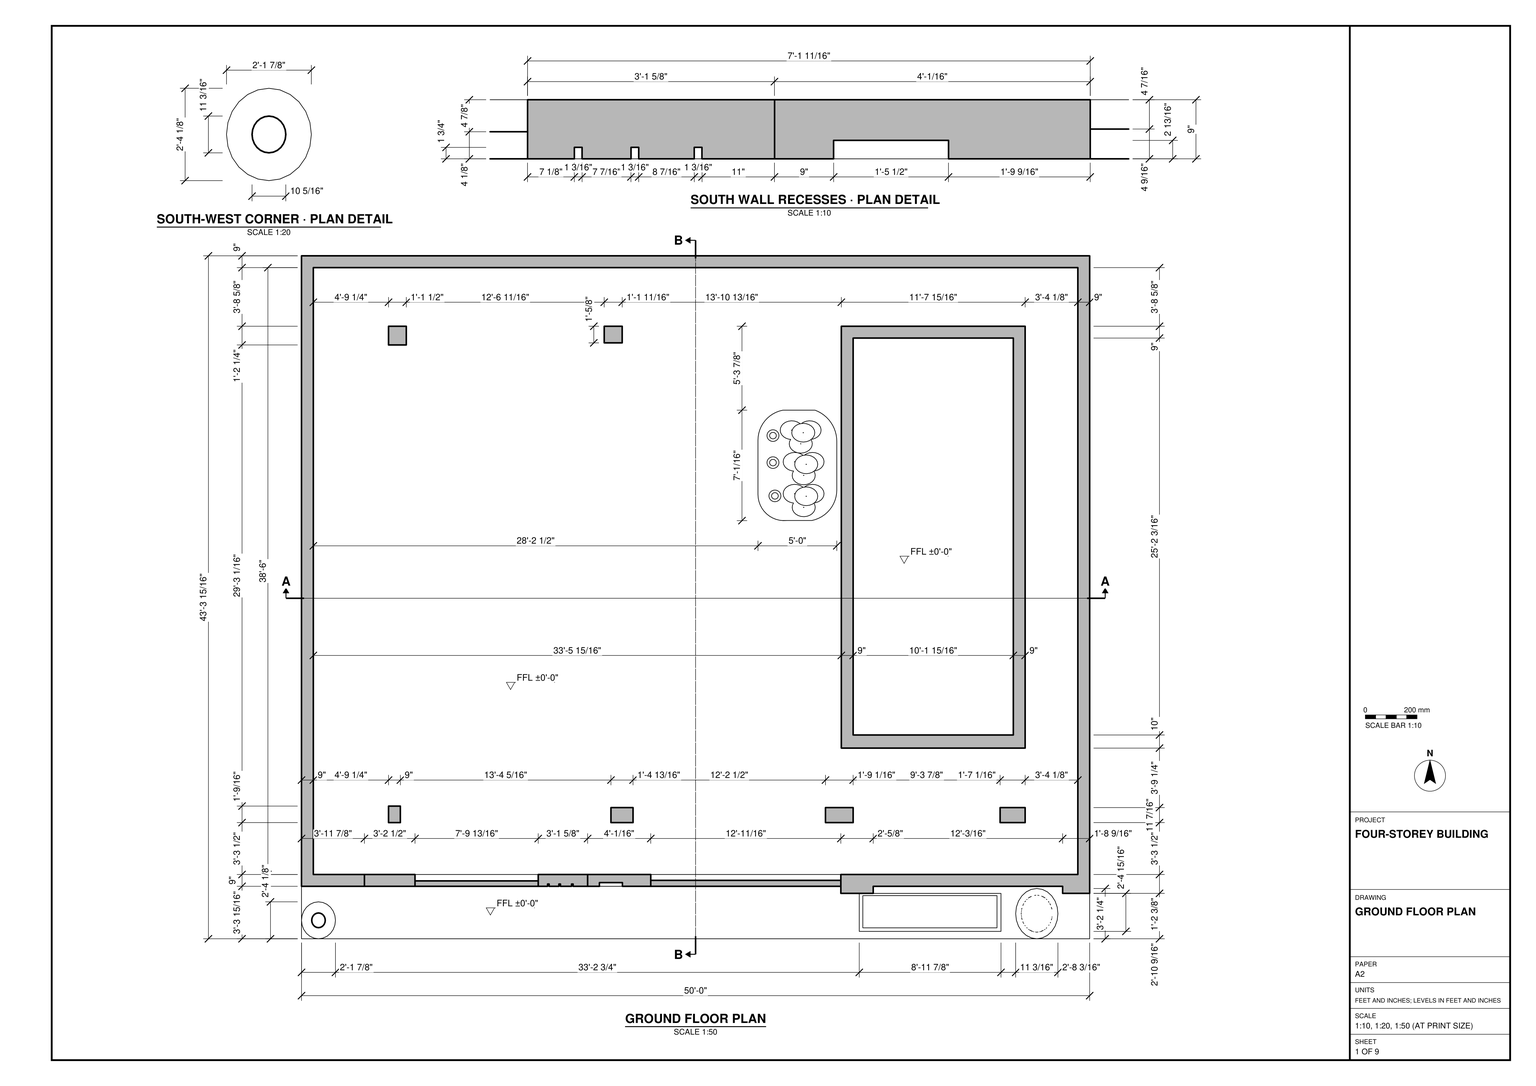
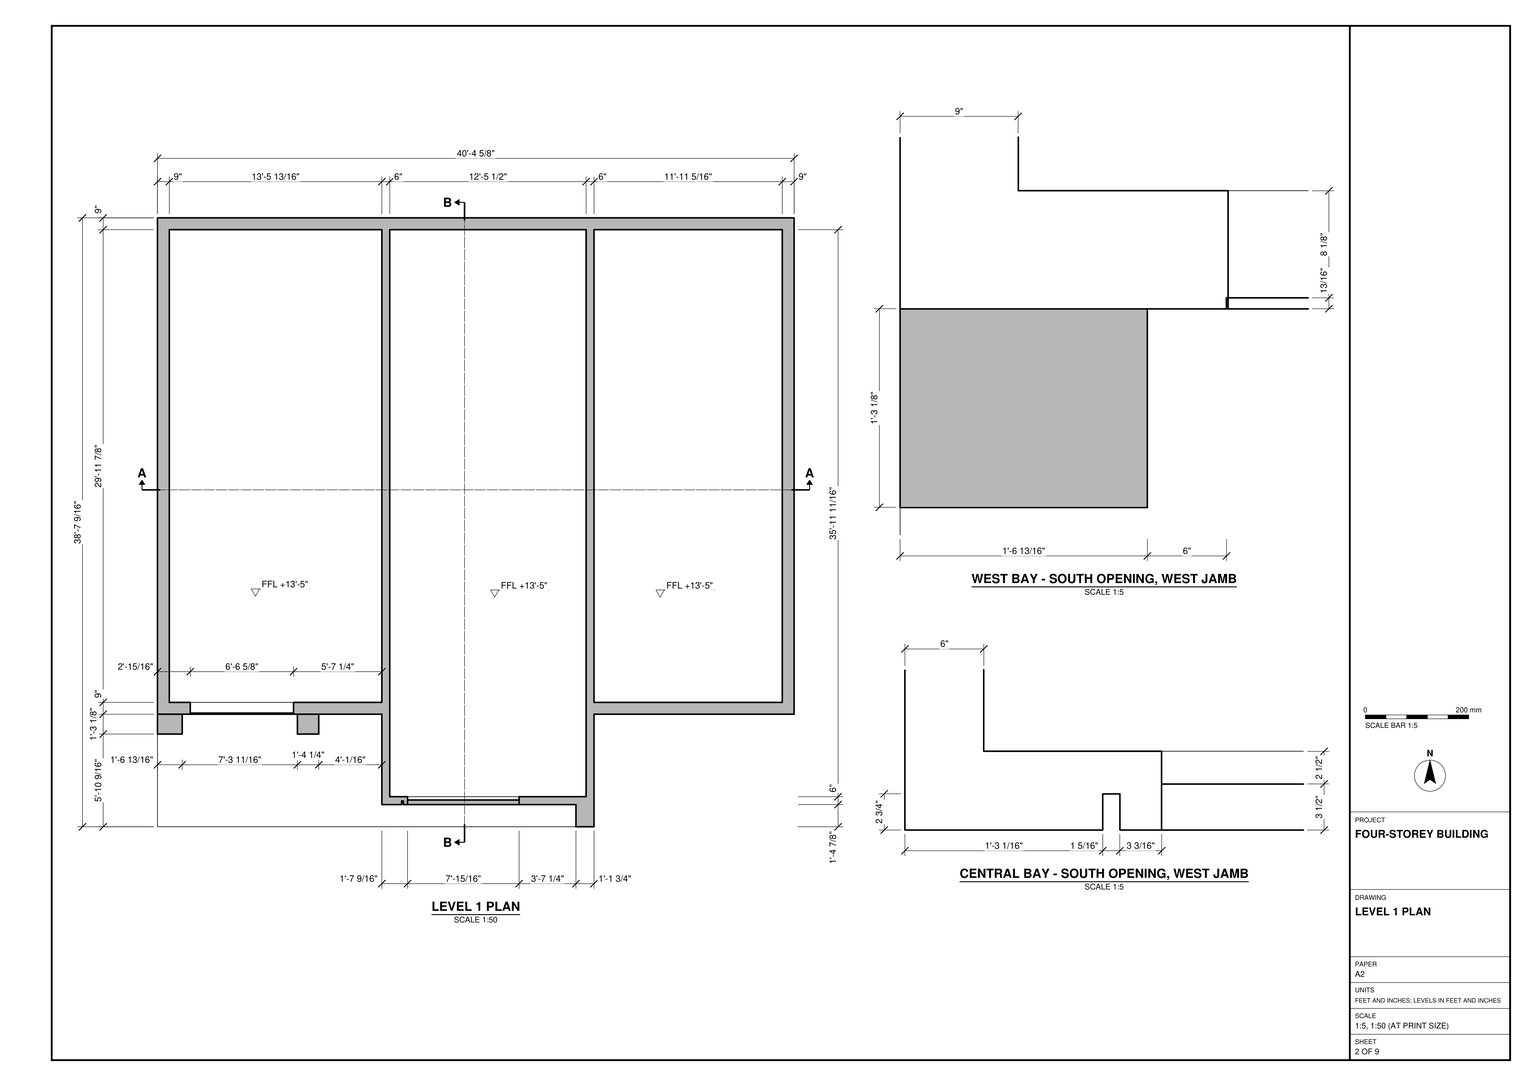
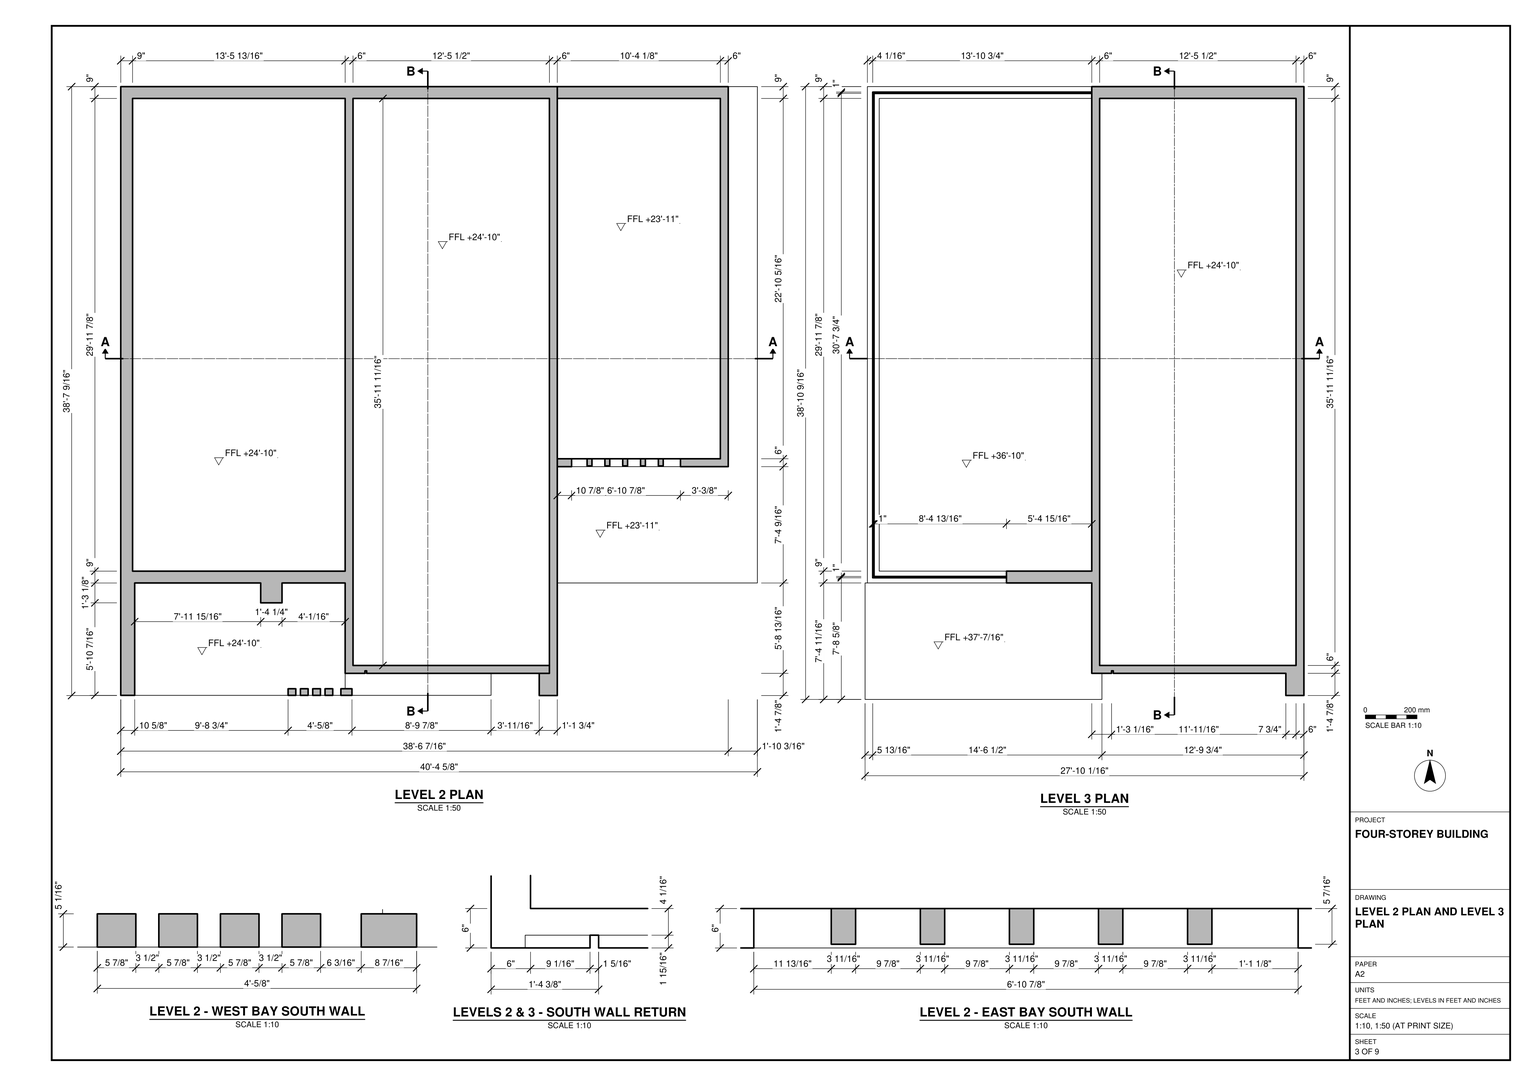
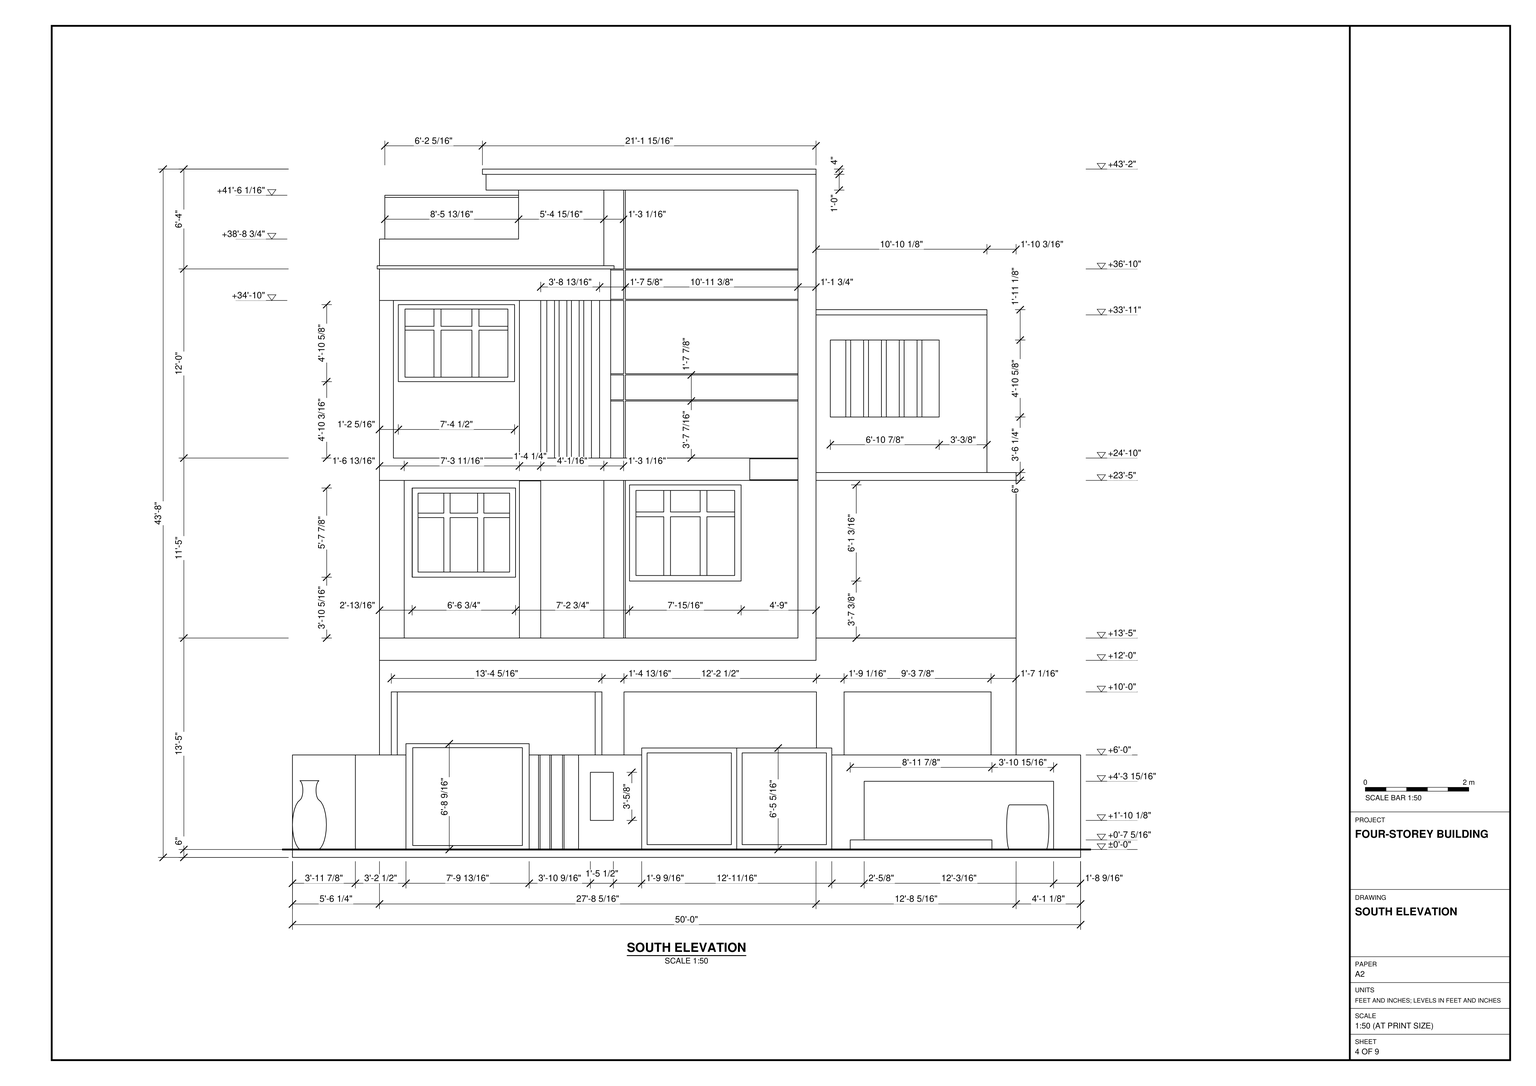
Build the four-storey building in SketchUp from task_files/diagram_01.pdf. Work in feet and inches. The overall size is 50'-0" east to west, 43'-5 7/16" north to south and 43'-8" high. Set the main floor levels at ±0'-0", +13'-5", +24'-10" and +36'-10". Follow the local changes in floor and roof height shown on the sheets rather than levelling each slab across all bays.

Lay out the largely open ground floor with its freestanding columns, long rectangular enclosure near the east side and narrow strip beyond the south wall. Use the plan details for the recesses in that wall. Above it, form the three north–south bays, with the central bay projecting farther south than the side bays. Follow the changes in footprint on the upper floors, including the setback of the east bay. Use the wall thicknesses shown, including the 9" perimeter walls and 6" dividing walls where dimensioned. Model the openings and jambs, floor slabs, exposed roof areas and roof edges from the plans and sections. Include stairs, built-in joinery and main furniture where shown.

Keep walls, slabs, roof elements and each furniture or joinery piece in separate groups or components. Use components for repeated parts. Decor and loose items may be any suitable library components. Save one SketchUp model as output_files/four_storey_building_with_stepped_upper_bays.skp.

# SketchUp Ruby script. Lengths in inches.
U = 1.inch
M = Sketchup.active_model
def pt(a) = Geom::Point3d.new(a.map { |v| v * U })
def face(e, loops, mat)
  f = e.add_face(loops[0].map { |a| pt(a) })
  loops[1..].each { |l| e.add_face(l.map { |a| pt(a) }).erase! }
  f.material = f.back_material = mat if mat
  f
end
# faces: each face lists its corners as indices into pts; further lists are holes
def faces(e, pts, list, mat = nil) = list.each { |f| face(e, (f[0].is_a?(Array) ? f : [f]).map { |l| l.map { |i| pts[i] } }, mat) }
# xy, xz, yz: faces in a plane at the given z, y or x. An outline is a flat list of corners, or four numbers for a rectangle; further outlines are holes
def ring(l) = l.size == 4 ? [[l[0], l[1]], [l[2], l[1]], [l[2], l[3]], [l[0], l[3]]] : l.each_slice(2).to_a
def flat(e, list, mat, &to3) = list.each { |f| face(e, (f[0].is_a?(Array) ? f : [f]).map { |l| ring(l).map { |u, v| to3.(u, v) } }, mat) }
def xy(e, z, list, mat = nil) = flat(e, list, mat) { |x, y| [x, y, z] }
def xz(e, y, list, mat = nil) = flat(e, list, mat) { |x, z| [x, y, z] }
def yz(e, x, list, mat = nil) = flat(e, list, mat) { |y, z| [x, y, z] }
def lines(e, pts, list) = list.each { |a, b| e.add_line(pt(pts[a]), pt(pts[b])) }
# prism: a flat outline (further loops are holes) pulled along v
def prism(e, loops, v, mat = nil)
  f = face(e, loops, mat); d = Geom::Vector3d.new(v.map { |x| x * U })
  f.pushpull(f.normal.samedirection?(d) ? d.length : -d.length)
end
def box(e, o, s, mat = nil) = prism(e, [[o, [o[0] + s[0], o[1], o[2]], [o[0] + s[0], o[1] + s[1], o[2]], [o[0], o[1] + s[1], o[2]]]], [0, 0, s[2]], mat)
def at(x, y, z, deg = 0) = Geom::Transformation.translation(pt([x, y, z])) * Geom::Transformation.rotation(ORIGIN, Z_AXIS, deg.degrees)
def axes(o, x, y, z) = Geom::Transformation.new([*x, 0, *y, 0, *z, 0, *pt(o).to_a, 1])
def part(name) = M.definitions.add(name)
# library, detail: a bought-in or finely detailed component or shape, given as its bounding box
def library(name, o, s) = part(name).tap { |d| box(d.entities, o, s) }
def detail(e, o, s) = box(e.add_group.entities, o, s)
def put(e, d, t, mat = nil) = e.add_instance(d, t).tap { |i| i.material = mat if mat }
def group(e, t, mat = nil) = e.add_group.tap { |g| g.transformation = t; g.material = mat if mat }.entities
root = M.entities
M.materials.add("[0056_Yellow]").color = [249, 242, 89]
M.materials.add("[0056_Yellow]1").color = [255, 255, 0]
M.materials.add("[0060_GrassGreen]").color = [62, 91, 76]
M.materials.add("[0073_MediumSeaGreen]").color = [60, 179, 113]
M.materials.add("[0111_SlateGray]").color = [120, 130, 144]
M.materials.add("[0123_DarkMagenta]").color = [145, 113, 139]
M.materials.add("[0124_Purple]").color = [128, 93, 128]
M.materials.add("[0131_Silver]").color = [192, 192, 192]
M.materials.add("[0136_Charcoal]").color = [35, 35, 35]
M.materials.add("[Brick Rough Tan]").color = [199, 186, 164]
M.materials.add("[Brick Rough Tan]1").color = [167, 141, 82]
M.materials.add("[Carrera Marble]").color = [207, 207, 207]
M.materials.add("[Color C08]").color = [102, 51, 0]
M.materials.add("[Color I01]").color = [204, 204, 255]
M.materials.add("[Color I06]").color = [0, 130, 204]
M.materials.add("[Color M00]").color = [255, 255, 255]
M.materials.add("[Color M01]").color = [226, 226, 226]
M.materials.add("[Color M02]").color = [198, 198, 198]
M.materials.add("[Color M03]").color = [170, 170, 170]
M.materials.add("[Color M04]").color = [142, 142, 142]
M.materials.add("[Color M06]").color = [86, 86, 86]
M.materials.add("[Color M07]").color = [58, 58, 58]
M.materials.add("[Concrete Block 8x8 Gray]").color = [157, 158, 154]
M.materials.add("[Concrete Block Retaining Gray]").color = [121, 121, 121]
M.materials.add("[Grass Dark Green]").color = [106, 157, 55]
M.materials.add("[Polished Concrete New]").color = [200, 200, 203]
M.materials.add("[Stone Flagstone Ashlar]").color = [106, 69, 26]
M.materials.add("[Translucent Glass Gray]").color = [128, 128, 128]
M.materials["[Translucent Glass Gray]"].alpha = 0.5
M.materials.add("[Wood Cherry Original]").color = [152, 86, 42]
M.materials.add("[Wood Floor Parquet]").color = [145, 89, 39]
c1 = part("Group\#1")
xy(c1.entities,0,[[0,0,56.875,3.5]],"[Wood Cherry Original]")
xy(c1.entities,3.27,[[3.27,0,17.44,3.5],[17.44,0,20.89,1.125],[20.89,0,36,3.5],[36,0,39.45,1.125],[39.45,0,53.6,3.5],
  [17.44,1.125,20.89,3.5],[36,1.125,39.45,3.5]],"[Wood Cherry Original]")
xy(c1.entities,38.03,[[3.27,1.125,17.44,3.5],[20.89,1.125,36,3.5],[39.45,1.125,53.6,3.5]],"[Wood Cherry Original]")
xy(c1.entities,40.86,[[3.27,1.125,17.44,3.5],[20.89,1.125,36,3.5],[39.45,1.125,53.6,3.5]],"[Wood Cherry Original]")
xy(c1.entities,53.6,[[3.27,0,17.44,3.5],[17.44,0,20.89,1.125],[20.89,0,36,3.5],[36,0,39.45,1.125],[39.45,0,53.6,3.5],
  [17.44,1.125,20.89,3.5],[36,1.125,39.45,3.5]],"[Wood Cherry Original]")
xy(c1.entities,56.875,[[0,0,56.875,3.5]],"[Wood Cherry Original]")
xz(c1.entities,0,[[[0,0,56.875,56.875],[3.27,3.27,53.6,53.6]]],"[Wood Cherry Original]")
xz(c1.entities,1.125,[[17.44,3.27,20.89,3.27,20.89,38.03,36,38.03,36,3.27,39.45,3.27,39.45,38.03,53.6,38.03,53.6,40.86,39.45,40.86,39.45,53.6,36,53.6,36,40.86,20.89,40.86,20.89,53.6,17.44,53.6,17.44,40.86,3.27,40.86,3.27,38.03,17.44,38.03]],"[Wood Cherry Original]")
xz(c1.entities,3.5,[[3.27,3.27,17.44,38.03],[20.89,3.27,36,38.03],[39.45,3.27,53.6,38.03],[3.27,40.86,17.44,53.6],[20.89,40.86,36,53.6],
  [39.45,40.86,53.6,53.6]],"[Translucent Glass Gray]")
xz(c1.entities,3.5,[[[0,0,56.875,56.875],[3.27,3.27,53.6,53.6]],[17.44,3.27,17.44,38.03,3.27,38.03,3.27,40.86,17.44,40.86,17.44,53.6,20.89,53.6,20.89,40.86,36,40.86,36,53.6,39.45,53.6,39.45,40.86,53.6,40.86,53.6,38.03,39.45,38.03,39.45,3.27,36,3.27,36,38.03,20.89,38.03,20.89,3.27]],"[Wood Cherry Original]")
yz(c1.entities,0,[[0,0,3.5,56.875]],"[Wood Cherry Original]")
yz(c1.entities,3.27,[[0,3.27,3.5,38.03],[0,38.03,1.125,40.86],[1.125,38.03,3.5,40.86],[0,40.86,3.5,53.6]],"[Wood Cherry Original]")
yz(c1.entities,17.44,[[1.125,3.27,3.5,38.03],[1.125,40.86,3.5,53.6]],"[Wood Cherry Original]")
yz(c1.entities,20.89,[[1.125,3.27,3.5,38.03],[1.125,40.86,3.5,53.6]],"[Wood Cherry Original]")
yz(c1.entities,36,[[1.125,3.27,3.5,38.03],[1.125,40.86,3.5,53.6]],"[Wood Cherry Original]")
yz(c1.entities,39.45,[[1.125,3.27,3.5,38.03],[1.125,40.86,3.5,53.6]],"[Wood Cherry Original]")
yz(c1.entities,53.6,[[0,3.27,3.5,38.03],[0,38.03,1.125,40.86],[1.125,38.03,3.5,40.86],[0,40.86,3.5,53.6]],"[Wood Cherry Original]")
yz(c1.entities,56.875,[[0,0,3.5,56.875]],"[Wood Cherry Original]")
c2 = library("Group\#4",[0,0,0],[25.84,28.11,66.36])
c3 = library("Group\#6",[0,0,0],[80.96,80.52,80.96])
c4 = library("Group\#7",[0,0,0],[79.77,94.6,79.77])
c5 = part("Group\#8")
xy(c5.entities,0,[[0.19,0.27,3.22,4.42]])
xy(c5.entities,14.6875,[[0,0,2.48,3.02]])
p = [[3.22,0.27,0],[2.48,0,14.6875],[0,0,14.6875],[0.19,0.27,0],[0,3.02,14.6875],[0.19,4.42,0],
  [3.22,4.42,0],[2.48,3.02,14.6875]]
faces(c5.entities,p,[[0,1,2,3],[2,4,5,3],[1,0,6,7],[5,4,7,6]])
c6 = library("Group\#10",[0,0,0],[17.53,14.22,10.22])
c7 = library("Group\#11",[0,0,0],[7.07,6.58,13.6])
xy(root,0,[[0,1.5,600,41.4375],[0,41.4375,600,521.4375]])
xy(root,6,[[410.58,36.0625,435.23,41.4375],[0,41.4375,0,521.4375,600,521.4375,600,41.4375,410.58,41.4375,410.58,50.4375,591,50.4375,591,512.4375,9,512.4375,9,50.4375,47.9,50.4375,47.9,41.4375],[47.9,41.4375,86.4,50.4375],[86.4,41.4375,180.2,50.4375],[180.2,41.4375,180.2,50.4375,217.8125,50.4375,217.8125,41.4375,206.75,41.4375,206.75,43.1875,205.58,43.1875,205.58,41.4375,197.125,41.4375,197.125,43.1875,195.95,43.1875,195.95,41.4375,188.5,41.4375,188.5,43.1875,187.33,43.1875,187.33,41.4375],
  [187.33,41.4375,188.5,43.1875],[195.95,41.4375,197.125,43.1875],[205.58,41.4375,206.75,43.1875],[217.8125,41.4375,265.875,50.4375],[265.875,41.4375,410.58,50.4375],
  [66.25,89.9375,75.25,102.51],[235.57,89.9375,252.38,101.375],[398.875,89.9375,419.9375,101.375],[531.8125,89.9375,550.875,101.375],[[410.9375,146.65,550.875,467.8125],[419.9375,156.63,541.875,458.8125]],
  [419.9375,156.63,541.875,458.8125],[66.25,453.5625,79.77,467.8125],[230.4375,455.17,244.125,467.8125]])
xy(root,6,[[579.41,36.0625,600,41.4375]],"[Color M04]")
xy(root,6,[[[424.6,7.12,532.48,36.05],[427.3125,9.83,529.45,34.34]]],"[Concrete Block Retaining Gray]")
xy(root,6,[[[0,1.5,600,1.5,600,36.0625,579.41,36.0625,579.41,41.4375,435.23,41.4375,435.23,36.0625,410.58,36.0625,410.58,41.4375,0,41.4375],[424.6,7.12,532.48,36.05]],[427.3125,9.83,529.45,34.34]],"[Grass Dark Green]")
xy(root,6,[[[9,50.4375,591,512.4375],[410.9375,146.65,550.875,467.8125],[398.875,89.9375,419.9375,101.375],[531.8125,89.9375,550.875,101.375],[66.25,453.5625,79.77,467.8125],[235.57,89.9375,252.38,101.375],[230.4375,455.17,244.125,467.8125],[66.25,89.9375,75.25,102.51]]],"[Polished Concrete New]")
xy(root,13.3125,[[[424.6,7.12,532.48,36.05],[427.3125,9.83,529.45,34.34]]],"[Concrete Block Retaining Gray]")
xy(root,28.15,[[226.8,41.4375,244.3,44.25]],"[Stone Flagstone Ashlar]")
xy(root,57.9375,[[435.23,36.0625,573.23,41.4375],[573.23,36.0625,579.41,41.4375]],"[Color M04]")
xy(root,64.78,[[226.8,41.4375,244.3,44.25]])
xy(root,78,[[180.2,41.4375,187.33,41.4375,187.33,43.1875,188.5,43.1875,188.5,41.4375,195.95,41.4375,195.95,43.1875,197.125,43.1875,197.125,41.4375,205.58,41.4375,205.58,43.1875,206.75,43.1875,206.75,41.4375,217.8125,41.4375,217.8125,50.4375,180.2,50.4375]],"[0060_GrassGreen]")
xy(root,78,[[410.58,36.0625,600,36.0625,600,521.4375,0,521.4375,0,41.4375,47.9,41.4375,47.9,50.4375,9,50.4375,9,512.4375,591,512.4375,591,50.4375,410.58,50.4375],[217.8125,41.4375,265.875,50.4375]],"[Color M04]")
xy(root,78,[[47.9,41.4375,86.4,50.4375]],"[Stone Flagstone Ashlar]")
xy(root,126,[[[410.9375,146.65,550.875,467.8125],[419.9375,156.63,541.875,458.8125]],[78.02,453.5625,79.77,455.17]])
xy(root,126,[[419.9375,89.9375,419.9375,101.375,398.875,101.375,398.875,98.9375,252.38,98.9375,252.38,101.375,235.57,101.375,235.57,98.9375,75.25,98.9375,75.25,102.51,410.9375,102.51,410.9375,146.65,550.875,146.65,550.875,101.375,531.8125,101.375,531.8125,89.9375],[75.25,89.9375,235.57,98.9375],[252.38,89.9375,398.875,98.9375],[66.25,102.51,78.02,453.5625],[79.77,455.17,230.4375,467.8125],
  [244.125,455.17,410.9375,467.8125]],"[Color M03]")
xy(root,144,[[78.02,102.51,410.9375,455.17]],"[Color M03]")
xy(root,146.4375,[[419.9375,156.63,541.875,458.8125]])
xy(root,150,[[75.25,98.9375,541.875,458.8125]])
xy(root,150,[[66.25,4.25,398.5625,89.9375]],"[0131_Silver]")
xy(root,167,[[66.25,4.25,384.8125,4.25,384.8125,21.125,253.43,21.125,253.43,23.875,252.12,23.875,252.12,21.125,237.0625,21.125,237.0625,89.9375,189.01,89.9375,189.01,74.8125,172.77,74.8125,172.77,89.9375,85.07,89.9375,85.07,74.8125,66.25,74.8125],[243.0625,27.125,392.5625,458.8125],[66.25,74.8125,85.07,89.9375],[172.77,74.8125,189.01,89.9375],[75.25,98.9375,237.0625,458.8125],
  [398.5625,98.9375,541.875,458.8125]])
xy(root,210.39,[[256.6,21.125,341.54,27.125]])
xy(root,213.33,[[91.22,89.9375,169.84,98.9375]])
xy(root,215,[[398.5625,98.9375,541.875,458.8125]])
xy(root,281.2,[[91.22,89.9375,169.84,98.9375]])
xy(root,283.58,[[256.6,21.125,341.54,27.125]])
xy(root,286.625,[[172.77,74.8125,189.01,89.9375]])
xy(root,287,[[237.0625,4.375,348.14,21.125],[252.12,21.125,253.43,23.875],[348.14,21.125,384.8125,21.5625],[66.25,74.8125,85.07,89.9375],[398.5625,89.9375,550.875,467.8125]])
xy(root,287,[[66.25,4.375,66.25,74.8125,85.07,74.8125,85.07,89.9375,237.0625,89.9375,237.0625,4.375]],"[0131_Silver]")
xy(root,287.48,[[348.14,21.125,384.8125,21.5625]])
xy(root,293,[[398.5625,178.5,398.5625,184.5,522.6875,184.5,522.6875,458.8125,398.5625,458.8125,398.5625,467.8125,528.6875,467.8125,528.6875,178.5],[398.5625,184.5,522.6875,458.8125]])
xy(root,293,[[398.5625,89.9375,550.875,89.9375,550.875,467.8125,528.6875,467.8125,528.6875,178.5,398.5625,178.5]],"[Color M06]")
xy(root,297.75,[[75.25,98.9375,237.0625,458.8125]])
xy(root,298,[[243.0625,27.125,392.5625,458.8125]])
xy(root,303.45,[[348.14,21.125,384.8125,22.25]])
xy(root,304,[[242.25,4.375,348.14,4.375,348.14,21.125,237.0625,21.125,237.0625,9.4375,242.25,9.4375],[348.14,21.125,384.8125,22.25],[243.0625,27.125,392.5625,458.8125],[172.77,74.8125,189.01,89.9375],[75.25,98.9375,237.0625,458.8125]])
xy(root,304,[[76.85,4.375,193.63,4.375,193.63,9.4375,199.5,9.4375,199.5,4.375,203,4.375,203,9.4375,208.88,9.4375,208.88,4.375,212.38,4.375,212.38,9.4375,218.25,9.4375,218.25,4.375,221.75,4.375,221.75,9.4375,227.63,9.4375,227.63,4.375,233.81,4.375,233.81,9.4375,237.0625,9.4375,237.0625,89.9375,189.01,89.9375,189.01,74.8125,172.77,74.8125,172.77,89.9375,76.85,89.9375]],"[0131_Silver]")
xy(root,304,[[252.12,21.125,253.43,23.0625]],"[Carrera Marble]")
xy(root,304,[[193.63,4.375,199.5,9.4375],[203,4.375,208.88,9.4375],[212.38,4.375,218.25,9.4375],[221.75,4.375,227.63,9.4375],[233.81,4.375,242.25,9.4375]],"[Color I01]")
xy(root,335.25,[[421.24,179.0625,424.95,184.5],[434.81,179.0625,438.51,184.5],[448.37,179.0625,452.08,184.5],[461.93,179.0625,465.64,184.5],[475.49,179.0625,479.2,184.5]])
xy(root,335.25,[[409.45,178.5,409.45,184.5,421.24,184.5,421.24,179.0625,424.95,179.0625,424.95,184.5,434.81,184.5,434.81,179.0625,438.51,179.0625,438.51,184.5,448.37,184.5,448.37,179.0625,452.08,179.0625,452.08,184.5,461.93,184.5,461.93,179.0625,465.64,179.0625,465.64,184.5,475.49,184.5,475.49,179.0625,479.2,179.0625,479.2,184.5,492.33,184.5,492.33,178.5]],"[0136_Charcoal]")
xy(root,347.4375,[[237.0625,21.125,252.12,23.0625],[253.43,21.125,384.8125,23.0625]],"[Carrera Marble]")
xy(root,348.35,[[237.0625,21.125,252.12,23.0625],[253.43,21.125,384.8125,23.0625]],"[Carrera Marble]")
xy(root,362.2,[[80.59,89.9375,169.09,98.9375]])
xy(root,367.3125,[[237.0625,21.125,252.12,23.0625],[253.43,21.125,384.8125,23.0625]],"[Carrera Marble]")
xy(root,368.22,[[237.0625,21.125,252.12,23.0625],[253.43,21.125,384.8125,23.0625]],"[Carrera Marble]")
xy(root,393.88,[[421.24,178.5,424.95,179.0625],[434.81,178.5,438.51,179.0625],[448.37,178.5,452.08,179.0625],[461.93,178.5,465.64,179.0625],[475.49,178.5,479.2,179.0625],
  [421.24,179.0625,424.95,184.5],[434.81,179.0625,438.51,184.5],[448.37,179.0625,452.08,184.5],[461.93,179.0625,465.64,184.5],[475.49,179.0625,479.2,184.5]])
xy(root,393.88,[[409.45,178.5,421.24,184.5],[424.95,178.5,434.81,184.5],[438.51,178.5,448.37,184.5],[452.08,178.5,461.93,184.5],[465.64,178.5,475.49,184.5],
  [479.2,178.5,492.33,184.5]],"[0136_Charcoal]")
xy(root,407,[[398.5625,184.5,522.6875,458.8125]])
xy(root,413,[[398.5625,178.5,528.6875,467.8125]])
xy(root,417,[[398.5625,178.5,528.6875,467.8125]],"[Color M07]")
xy(root,420.83,[[80.59,89.9375,169.09,98.9375]])
xy(root,424,[[76.85,4.375,76.85,89.9375,172.77,89.9375,172.77,74.8125,189.01,74.8125,189.01,89.9375,237.0625,89.9375,237.0625,21.125,242.25,21.125,242.25,9.4375,233.81,9.4375,233.81,4.375,227.63,4.375,227.63,9.4375,221.75,9.4375,221.75,4.375,218.25,4.375,218.25,9.4375,212.38,9.4375,212.38,4.375,208.88,4.375,208.88,9.4375,203,9.4375,203,4.375,199.5,4.375,199.5,9.4375,193.63,9.4375,193.63,4.375]],"[0131_Silver]")
xy(root,424,[[242.25,21.125,252.12,23.0625],[253.43,21.125,384.8125,23.0625]],"[Carrera Marble]")
xy(root,424.91,[[242.25,21.125,252.12,23.0625],[253.43,21.125,384.8125,23.0625]],"[Carrera Marble]")
xy(root,436,[[75.25,98.9375,237.0625,458.8125]])
xy(root,447.16,[[242.25,21.125,252.12,23.0625],[253.43,21.125,384.8125,23.0625]],"[Carrera Marble]")
xy(root,448,[[66.25,4.375,66.25,89.9375,237.0625,89.9375,237.0625,21.125,242.25,21.125,242.25,4.375],[75.25,98.9375,237.0625,458.8125]])
xy(root,448,[[242.25,21.125,252.12,23.0625],[253.43,21.125,384.8125,23.0625]],"[Carrera Marble]")
xy(root,448,[[64.5,1.25,64.5,89.9375,66.25,89.9375,66.25,4.375,242.25,4.375,242.25,21.125,244.8125,21.125,244.8125,1.25]],"[Color M07]")
xy(root,450.4375,[[64.5,1.25,244.8125,1.25,244.8125,21.125,237.0625,21.125,237.0625,89.9375,64.5,89.9375]],"[Color M07]")
xy(root,470.75,[[70.3125,93.875,70.3125,463.625,237.0625,463.625,237.0625,462.625,71.3125,462.625,71.3125,94.875,172.125,94.875,172.125,93.875]])
xy(root,470.75,[[66.25,89.9375,172.125,89.9375,172.125,93.875,70.3125,93.875,70.3125,463.625,237.0625,463.625,237.0625,467.8125,66.25,467.8125],[71.3125,94.875,172.125,94.875,172.125,98.9375,75.25,98.9375,75.25,458.8125,237.0625,458.8125,237.0625,462.625,71.3125,462.625]],"[0124_Purple]")
xy(root,496,[[243.0625,27.125,392.5625,458.8125]])
xy(root,502.4375,[[70.3125,93.875,70.3125,463.625,237.0625,463.625,237.0625,462.625,71.3125,462.625,71.3125,94.875,172.125,94.875,172.125,93.875]])
xy(root,504.0625,[[70.3125,93.875,172.125,93.875,172.125,94.875,71.3125,94.875,71.3125,462.625,237.0625,462.625,237.0625,463.625,70.3125,463.625]])
xy(root,508,[[147.375,4.25,147.375,98.9375,172.125,98.9375,172.125,89.9375,237.0625,89.9375,237.0625,21.125,252.12,21.125,252.12,23.0625,253.43,23.0625,253.43,21.125,384.8125,21.125,384.8125,4.25],[147.375,98.9375,237.0625,467.8125]])
xy(root,520,[[147.375,4.25,398.5625,467.8125]])
xy(root,520,[[144.625,0,144.625,467.8125,147.375,467.8125,147.375,4.25,398.5625,4.25,398.5625,0]],"[0136_Charcoal]")
xy(root,524,[[144.625,0,398.5625,467.8125]],"[0136_Charcoal]")
xz(root,0,[[144.625,520,398.5625,524]],"[0136_Charcoal]")
xz(root,1.25,[[64.5,448,244.8125,450.4375]],"[Color M07]")
xz(root,1.5,[[0,0,600,6]])
xz(root,4.25,[[66.25,150,398.5625,150,398.5625,520,147.375,520,147.375,508,384.8125,508,384.8125,167,66.25,167]],"[0131_Silver]")
xz(root,4.375,[[66.25,424,242.25,448]])
xz(root,4.375,[[66.25,287,348.14,287,348.14,304,76.85,304,76.85,424,66.25,424]],"[0131_Silver]")
xz(root,4.375,[[193.63,304,199.5,424],[203,304,208.88,424],[212.38,304,218.25,424],[221.75,304,227.63,424],[233.81,304,242.25,424]],"[Color I01]")
xz(root,7.12,[[424.6,6,532.48,13.3125]],"[Concrete Block Retaining Gray]")
xz(root,9.4375,[[193.63,304,199.5,424],[203,304,208.88,424],[212.38,304,218.25,424],[221.75,304,227.63,424],[233.81,304,242.25,424]],"[Color I01]")
xz(root,9.83,[[427.3125,6,529.45,13.3125]],"[Concrete Block Retaining Gray]")
xz(root,21.125,[[252.12,287,253.43,304],[253.43,287,348.14,304],[384.8125,287,392.5625,304],[384.8125,304,392.5625,424],[384.8125,424,392.5625,448],
  [237.0625,448,244.8125,450.4375]])
xz(root,21.125,[[237.0625,167,252.12,287],[[253.43,167,384.8125,287],[256.6,210.39,341.54,283.58]],[348.14,287.48,384.8125,303.45],[237.0625,304,252.12,347.4375],[253.43,304,384.8125,347.4375],
  [237.0625,348.35,252.12,367.3125],[253.43,348.35,384.8125,367.3125],[237.0625,368.22,252.12,424],[253.43,368.22,384.8125,424],[242.25,424.91,252.12,447.16],
  [253.43,424.91,384.8125,447.16],[244.8125,448,252.12,448,252.12,508,237.0625,508,237.0625,450.4375,244.8125,450.4375],[253.43,448,384.8125,508]],"[Carrera Marble]")
xz(root,21.5625,[[348.14,287,384.8125,287.48]],"[Carrera Marble]")
xz(root,22.25,[[348.14,303.45,384.8125,304]],"[Carrera Marble]")
xz(root,23.0625,[[252.12,304,253.43,304,253.43,347.4375,384.8125,347.4375,384.8125,348.35,253.43,348.35,253.43,367.3125,384.8125,367.3125,384.8125,368.22,253.43,368.22,253.43,424,384.8125,424,384.8125,424.91,253.43,424.91,253.43,447.16,384.8125,447.16,384.8125,448,253.43,448,253.43,508,252.12,508,252.12,448,242.25,448,242.25,447.16,252.12,447.16,252.12,424.91,242.25,424.91,242.25,424,252.12,424,252.12,368.22,237.0625,368.22,237.0625,367.3125,252.12,367.3125,252.12,348.35,237.0625,348.35,237.0625,347.4375,252.12,347.4375]],"[Carrera Marble]")
xz(root,23.875,[[252.12,167,253.43,287]])
xz(root,27.125,[[[243.0625,167,392.5625,287],[256.6,210.39,341.54,283.58]],[243.0625,287,392.5625,298],[243.0625,298,392.5625,304],[243.0625,304,392.5625,424],[243.0625,424,392.5625,448],
  [243.0625,448,392.5625,496]])
xz(root,34.34,[[427.3125,6,529.45,13.3125]],"[Concrete Block Retaining Gray]")
xz(root,36.05,[[424.6,6,532.48,13.3125]],"[Concrete Block Retaining Gray]")
xz(root,36.0625,[[410.58,6,435.23,6,435.23,57.9375,579.41,57.9375,579.41,6,600,6,600,78,410.58,78]],"[Color M04]")
xz(root,41.4375,[[0,0,600,6],[0,6,47.9,78]])
xz(root,41.4375,[[180.2,6,187.33,78],[188.5,6,195.95,78],[197.125,6,205.58,78],[206.75,6,217.8125,78]],"[0060_GrassGreen]")
xz(root,41.4375,[[435.23,6,579.41,57.9375]],"[Brick Rough Tan]1")
xz(root,41.4375,[[[217.8125,6,265.875,78],[226.8,28.15,244.3,64.78]]],"[Color M04]")
xz(root,41.4375,[[47.9,6,86.4,78]],"[Stone Flagstone Ashlar]")
xz(root,43.1875,[[187.33,6,188.5,78],[195.95,6,197.125,78],[205.58,6,206.75,78]],"[0056_Yellow]")
xz(root,44.25,[[226.8,28.15,244.3,64.78]],"[Stone Flagstone Ashlar]")
xz(root,50.4375,[[9,6,47.9,78]])
xz(root,50.4375,[[180.2,6,217.8125,78]],"[0060_GrassGreen]")
xz(root,50.4375,[[217.8125,6,265.875,78],[410.58,6,591,78]],"[Color M04]")
xz(root,50.4375,[[47.9,6,86.4,78]],"[Stone Flagstone Ashlar]")
xz(root,74.8125,[[66.25,167,85.07,287],[172.77,167,189.01,286.625],[172.77,304,189.01,424]],"[0111_SlateGray]")
xz(root,89.9375,[[172.77,166.625,189.01,167],[66.25,167,85.07,287],[172.77,167,189.01,286.625],[66.25,448,237.0625,450.4375]])
xz(root,89.9375,[[189.01,304,237.0625,424],[66.25,450.4375,237.0625,450.4375,237.0625,508,172.125,508,172.125,470.75,66.25,470.75]],"[0123_DarkMagenta]")
xz(root,89.9375,[[[85.07,167,172.77,167,172.77,286.625,189.01,286.625,189.01,167,237.0625,167,237.0625,287,85.07,287],[91.22,213.33,169.84,281.2]],[[76.85,304,172.77,424],[80.59,362.2,169.09,420.83]]],"[Brick Rough Tan]")
xz(root,89.9375,[[66.25,6,75.25,6,75.25,126,235.57,126,235.57,6,252.38,6,252.38,126,398.875,126,398.875,6,419.9375,6,419.9375,126,531.8125,126,531.8125,6,550.875,6,550.875,167,398.5625,167,398.5625,150,66.25,150]],"[Color M01]")
xz(root,89.9375,[[398.5625,287,550.875,293]],"[Color M06]")
xz(root,89.9375,[[64.5,448,66.25,450.4375]],"[Color M07]")
xz(root,89.9375,[[398.5625,167,550.875,287]],"[Concrete Block 8x8 Gray]")
xz(root,93.875,[[70.3125,502.4375,172.125,504.0625]])
xz(root,93.875,[[70.3125,470.75,172.125,502.4375]],"[Translucent Glass Gray]")
xz(root,94.875,[[71.3125,502.4375,172.125,504.0625]])
xz(root,94.875,[[71.3125,470.75,172.125,502.4375]],"[Translucent Glass Gray]")
xz(root,98.9375,[[[75.25,167,237.0625,287],[91.22,213.33,169.84,281.2]],[398.5625,167,541.875,215],[75.25,287,237.0625,297.75],[75.25,297.75,172.125,304],[172.125,297.75,192.91,304],
  [192.91,297.75,237.0625,304],[[75.25,304,237.0625,424],[80.59,362.2,169.09,420.83]],[75.25,424,237.0625,436],[75.25,436,172.125,448],[172.125,436,220.3125,448],
  [220.3125,436,237.0625,448],[75.25,448,172.125,470.75],[172.125,448,237.0625,508]])
xz(root,101.375,[[235.57,6,252.38,126],[398.875,6,419.9375,126],[531.8125,6,550.875,126]])
xz(root,102.51,[[66.25,6,75.25,126],[78.02,126,410.9375,144]],"[Color M03]")
xz(root,146.65,[[410.9375,6,550.875,126]],"[Color M03]")
xz(root,156.63,[[419.9375,6,541.875,126],[419.9375,126,541.875,146.4375]])
xz(root,178.5,[[[398.5625,293,528.6875,413],[409.45,335.25,492.33,393.88]]],"[Color M02]")
xz(root,178.5,[[398.5625,413,528.6875,417]],"[Color M07]")
xz(root,179.0625,[[421.24,335.25,424.95,393.88],[448.37,335.25,452.08,393.88],[461.93,335.25,465.64,393.88],[475.49,335.25,479.2,393.88]])
xz(root,179.0625,[[434.81,335.25,438.51,393.88]],"[Color M00]")
xz(root,184.5,[[[398.5625,293,522.6875,407],[409.45,335.25,492.33,393.88]],[421.24,335.25,424.95,393.88],[434.81,335.25,438.51,393.88],[448.37,335.25,452.08,393.88],[461.93,335.25,465.64,393.88],
  [475.49,335.25,479.2,393.88]])
xz(root,184.5,[[409.45,335.25,421.24,393.88],[424.95,335.25,434.81,393.88],[438.51,335.25,448.37,393.88],[452.08,335.25,461.93,393.88],[465.64,335.25,475.49,393.88],
  [479.2,335.25,492.33,393.88]],"[Translucent Glass Gray]")
xz(root,453.5625,[[66.25,6,79.77,126]],"[Color M03]")
xz(root,455.17,[[230.4375,6,244.125,126],[78.02,126,410.9375,144]],"[Color M03]")
xz(root,458.8125,[[419.9375,6,541.875,126],[419.9375,126,541.875,146.4375],[419.9375,146.4375,541.875,150],[419.9375,150,541.875,167],[75.25,167,237.0625,287],
  [243.0625,167,392.5625,287],[398.5625,167,419.9375,215],[419.9375,167,541.875,215],[75.25,287,237.0625,297.75],[243.0625,287,392.5625,298],
  [398.5625,293,522.6875,407],[75.25,297.75,237.0625,304],[243.0625,298,392.5625,304],[75.25,304,237.0625,424],[243.0625,304,392.5625,424],
  [75.25,424,237.0625,436],[243.0625,424,392.5625,448],[75.25,436,237.0625,448],[75.25,448,237.0625,470.75],[243.0625,448,392.5625,496]])
xz(root,462.625,[[71.3125,502.4375,237.0625,504.0625]])
xz(root,462.625,[[71.3125,470.75,237.0625,502.4375]],"[Translucent Glass Gray]")
xz(root,463.625,[[70.3125,502.4375,237.0625,504.0625]])
xz(root,463.625,[[70.3125,470.75,237.0625,502.4375]],"[Translucent Glass Gray]")
xz(root,467.8125,[[147.375,508,398.5625,520]])
xz(root,467.8125,[[66.25,448,66.25,470.75,237.0625,470.75,237.0625,508,398.5625,508,398.5625,448]],"[0123_DarkMagenta]")
xz(root,467.8125,[[144.625,520,398.5625,524]],"[0136_Charcoal]")
xz(root,467.8125,[[66.25,150,66.25,448,398.5625,448,398.5625,287,550.875,287,550.875,150],[398.5625,293,528.6875,413]],"[Color M02]")
xz(root,467.8125,[[66.25,6,66.25,150,550.875,150,550.875,126,244.125,126,244.125,6,230.4375,6,230.4375,126,79.77,126,79.77,6],[410.9375,6,550.875,126]],"[Color M03]")
xz(root,467.8125,[[398.5625,287,550.875,293]],"[Color M06]")
xz(root,467.8125,[[398.5625,413,528.6875,417]],"[Color M07]")
xz(root,512.4375,[[9,6,591,78]])
xz(root,521.4375,[[0,0,600,6],[0,6,600,78]])
yz(root,0,[[1.5,0,41.4375,6],[41.4375,0,521.4375,6],[41.4375,6,521.4375,78]])
yz(root,9,[[50.4375,6,512.4375,78]])
yz(root,47.9,[[41.4375,6,50.4375,78]])
yz(root,64.5,[[1.25,448,89.9375,450.4375]],"[Color M07]")
yz(root,66.25,[[74.8125,167,89.9375,287]],"[0111_SlateGray]")
yz(root,66.25,[[89.9375,448,467.8125,470.75]],"[0123_DarkMagenta]")
yz(root,66.25,[[4.25,150,89.9375,167]],"[0131_Silver]")
yz(root,66.25,[[89.9375,150,89.9375,287,4.375,287,4.375,448,467.8125,448,467.8125,150]],"[Color M02]")
yz(root,66.25,[[89.9375,6,89.9375,150,467.8125,150,467.8125,6,453.5625,6,453.5625,126,102.51,126,102.51,6]],"[Color M03]")
yz(root,70.3125,[[93.875,502.4375,463.625,504.0625]])
yz(root,70.3125,[[93.875,470.75,463.625,502.4375]],"[Translucent Glass Gray]")
yz(root,71.3125,[[94.875,502.4375,462.625,504.0625]])
yz(root,71.3125,[[94.875,470.75,462.625,502.4375]],"[Translucent Glass Gray]")
yz(root,75.25,[[98.9375,150,458.8125,167],[98.9375,167,458.8125,287],[98.9375,287,458.8125,297.75],[98.9375,297.75,458.8125,304],[98.9375,304,458.8125,424],
  [98.9375,424,458.8125,436],[98.9375,436,458.8125,448],[98.9375,448,458.8125,470.75]])
yz(root,75.25,[[89.9375,6,102.51,126]],"[Color M03]")
yz(root,76.85,[[4.375,304,89.9375,424]])
yz(root,78.02,[[102.51,126,455.17,144]],"[Color M03]")
yz(root,79.77,[[453.5625,6,467.8125,126]],"[Color M03]")
yz(root,80.59,[[89.9375,362.2,98.9375,420.83]])
yz(root,85.07,[[74.8125,286.625,89.9375,287]])
yz(root,85.07,[[74.8125,167,89.9375,286.625]],"[0111_SlateGray]")
yz(root,86.4,[[41.4375,6,50.4375,78]],"[Stone Flagstone Ashlar]")
yz(root,91.22,[[89.9375,213.33,98.9375,281.2]])
yz(root,144.625,[[0,520,467.8125,524]],"[0136_Charcoal]")
yz(root,147.375,[[4.25,508,467.8125,520]])
yz(root,169.09,[[89.9375,362.2,98.9375,420.83]])
yz(root,169.84,[[89.9375,213.33,98.9375,281.2]])
yz(root,172.125,[[93.875,470.75,94.875,502.4375],[93.875,502.4375,94.875,504.0625]])
yz(root,172.125,[[89.9375,470.75,89.9375,508,98.9375,508,98.9375,470.75,94.875,470.75,94.875,504.0625,93.875,504.0625,93.875,470.75]],"[0124_Purple]")
yz(root,172.77,[[74.8125,167,89.9375,286.625],[74.8125,304,89.9375,424]],"[0111_SlateGray]")
yz(root,180.2,[[41.4375,6,50.4375,78]],"[0060_GrassGreen]")
yz(root,187.33,[[41.4375,6,43.1875,78]],"[0056_Yellow]")
yz(root,188.5,[[41.4375,6,43.1875,78]],"[0056_Yellow]")
yz(root,189.01,[[74.8125,167,89.9375,286.625],[74.8125,304,89.9375,424]],"[0111_SlateGray]")
yz(root,193.63,[[4.375,304,9.4375,424]],"[Color I01]")
yz(root,195.95,[[41.4375,6,43.1875,78]],"[0056_Yellow]")
yz(root,197.125,[[41.4375,6,43.1875,78]],"[0056_Yellow]")
yz(root,199.5,[[4.375,304,9.4375,424]],"[Color I01]")
yz(root,203,[[4.375,304,9.4375,424]],"[Color I01]")
yz(root,205.58,[[41.4375,6,43.1875,78]],"[0056_Yellow]")
yz(root,206.75,[[41.4375,6,43.1875,78]],"[0056_Yellow]")
yz(root,208.88,[[4.375,304,9.4375,424]],"[Color I01]")
yz(root,212.38,[[4.375,304,9.4375,424]],"[Color I01]")
yz(root,217.8125,[[41.4375,6,50.4375,78]])
yz(root,218.25,[[4.375,304,9.4375,424]],"[Color I01]")
yz(root,221.75,[[4.375,304,9.4375,424]],"[Color I01]")
yz(root,226.8,[[41.4375,28.15,44.25,64.78]],"[0056_Yellow]1")
yz(root,227.63,[[4.375,304,9.4375,424]],"[Color I01]")
yz(root,230.4375,[[455.17,6,467.8125,126]])
yz(root,233.81,[[4.375,304,9.4375,424]],"[Color I01]")
yz(root,235.57,[[89.9375,6,101.375,126]],"[Color M03]")
yz(root,237.0625,[[98.9375,167,458.8125,287],[98.9375,287,458.8125,297.75],[98.9375,297.75,458.8125,304],[98.9375,304,458.8125,424],[98.9375,424,458.8125,436],
  [98.9375,436,458.8125,448],[21.125,448,89.9375,450.4375],[462.625,470.75,463.625,502.4375],[462.625,502.4375,463.625,504.0625]])
yz(root,237.0625,[[458.8125,470.75,458.8125,508,467.8125,508,467.8125,470.75,463.625,470.75,463.625,504.0625,462.625,504.0625,462.625,470.75]],"[0124_Purple]")
yz(root,237.0625,[[21.125,167,89.9375,287],[21.125,304,21.125,347.4375,23.0625,347.4375,23.0625,348.35,21.125,348.35,21.125,367.3125,23.0625,367.3125,23.0625,368.22,21.125,368.22,21.125,424,89.9375,424,89.9375,304],[21.125,450.4375,89.9375,508]],"[Carrera Marble]")
yz(root,237.0625,[[98.9375,448,458.8125,508]],"[Color M02]")
yz(root,242.25,[[4.375,424,23.0625,424,23.0625,424.91,21.125,424.91,21.125,447.16,23.0625,447.16,23.0625,448,4.375,448]])
yz(root,242.25,[[4.375,304,9.4375,424]],"[Color I01]")
yz(root,243.0625,[[27.125,167,458.8125,287],[27.125,287,458.8125,298],[27.125,298,125.29,304],[125.29,298,162.91,304],[162.91,298,458.8125,304],
  [27.125,304,458.8125,424],[27.125,424,458.8125,448],[27.125,448,458.8125,496]])
yz(root,244.125,[[455.17,6,467.8125,126]],"[Color M03]")
yz(root,244.3,[[41.4375,28.15,44.25,64.78]],"[Stone Flagstone Ashlar]")
yz(root,244.8125,[[1.25,448,21.125,450.4375]],"[Color M07]")
yz(root,252.12,[[21.125,167,23.875,287]])
yz(root,252.12,[[21.125,304,23.0625,347.4375],[21.125,348.35,23.0625,367.3125],[21.125,368.22,23.0625,424],[21.125,424.91,23.0625,447.16],[21.125,448,23.0625,508]],"[Carrera Marble]")
yz(root,252.38,[[89.9375,6,101.375,126]],"[Color M03]")
yz(root,253.43,[[21.125,167,23.875,287]])
yz(root,253.43,[[21.125,304,23.0625,347.4375],[21.125,348.35,23.0625,367.3125],[21.125,368.22,23.0625,424],[21.125,424.91,23.0625,447.16],[21.125,448,23.0625,508]],"[Carrera Marble]")
yz(root,256.6,[[21.125,210.39,27.125,283.58]])
yz(root,265.875,[[41.4375,6,50.4375,78]],"[Color M04]")
yz(root,341.54,[[21.125,210.39,27.125,283.58]])
yz(root,348.14,[[4.375,287,21.125,304],[21.125,287,21.5625,287.48],[21.125,303.45,22.25,304]])
yz(root,384.8125,[[4.25,167,21.125,508],[21.125,287,21.5625,287.48],[21.125,303.45,22.25,304]])
yz(root,384.8125,[[21.125,347.4375,23.0625,348.35],[21.125,367.3125,23.0625,368.22],[21.125,424,23.0625,424.91],[21.125,447.16,23.0625,448]],"[Carrera Marble]")
yz(root,392.5625,[[27.125,167,458.8125,287],[21.125,287,27.125,304],[27.125,287,458.8125,298],[27.125,298,458.8125,304],[21.125,304,27.125,424],
  [27.125,304,458.8125,424],[21.125,424,27.125,448],[27.125,424,458.8125,448],[27.125,448,458.8125,496]])
yz(root,398.5625,[[98.9375,167,458.8125,215],[98.9375,215,458.8125,287],[89.9375,287,98.9375,293],[98.9375,287,458.8125,293],[458.8125,287,467.8125,293],
  [178.5,293,184.5,304],[184.5,293,458.8125,304],[458.8125,293,467.8125,304],[178.5,304,184.5,413],[184.5,304,458.8125,407],
  [458.8125,304,467.8125,413],[184.5,407,458.8125,413],[178.5,413,184.5,417],[184.5,413,458.8125,417],[458.8125,413,467.8125,417]])
yz(root,398.5625,[[0,520,467.8125,524]],"[0136_Charcoal]")
yz(root,398.5625,[[4.25,150,89.9375,150,89.9375,293,178.5,293,178.5,417,467.8125,417,467.8125,520,4.25,520]],"[Color M02]")
yz(root,398.875,[[89.9375,6,101.375,126]],"[Color M03]")
yz(root,409.45,[[178.5,335.25,184.5,393.88]],"[0136_Charcoal]")
yz(root,410.58,[[36.0625,6,50.4375,78]],"[Color M04]")
yz(root,410.9375,[[146.65,6,467.8125,126],[102.51,126,455.17,144]],"[Color M03]")
yz(root,419.9375,[[156.63,6,458.8125,126],[156.63,126,458.8125,146.4375]])
yz(root,419.9375,[[89.9375,6,101.375,126]],"[Color M03]")
yz(root,421.24,[[179.0625,335.25,184.5,393.88]])
yz(root,424.6,[[7.12,6,36.05,13.3125]],"[Concrete Block Retaining Gray]")
yz(root,424.95,[[179.0625,335.25,184.5,393.88]])
yz(root,427.3125,[[9.83,6,34.34,13.3125]],"[Concrete Block Retaining Gray]")
yz(root,434.81,[[179.0625,335.25,184.5,393.88]])
yz(root,435.23,[[36.0625,6,41.4375,57.9375]],"[Color M04]")
yz(root,438.51,[[179.0625,335.25,184.5,393.88]])
yz(root,448.37,[[179.0625,335.25,184.5,393.88]])
yz(root,452.08,[[179.0625,335.25,184.5,393.88]])
yz(root,461.93,[[179.0625,335.25,184.5,393.88]])
yz(root,465.64,[[179.0625,335.25,184.5,393.88]])
yz(root,475.49,[[179.0625,335.25,184.5,393.88]])
yz(root,479.2,[[179.0625,335.25,184.5,393.88]])
yz(root,492.33,[[178.5,335.25,184.5,393.88]],"[0136_Charcoal]")
yz(root,522.6875,[[184.5,293,458.8125,407]])
yz(root,528.6875,[[178.5,293,467.8125,413]],"[Color M02]")
yz(root,528.6875,[[178.5,413,467.8125,417]],"[Color M07]")
yz(root,529.45,[[9.83,6,34.34,13.3125]],"[Concrete Block Retaining Gray]")
yz(root,531.8125,[[89.9375,6,101.375,126]],"[Color M03]")
yz(root,532.48,[[7.12,6,36.05,13.3125]],"[Concrete Block Retaining Gray]")
yz(root,541.875,[[156.63,6,458.8125,126],[156.63,126,458.8125,146.4375],[156.63,146.4375,458.8125,150],[98.9375,150,156.63,167],[156.63,150,458.8125,167],
  [98.9375,167,156.63,215],[156.63,167,458.8125,215]])
yz(root,550.875,[[89.9375,6,101.375,126],[146.65,6,467.8125,126],[89.9375,126,467.8125,167],[89.9375,167,467.8125,287]],"[Color M03]")
yz(root,550.875,[[89.9375,287,467.8125,293]],"[Color M06]")
yz(root,579.41,[[36.0625,6,41.4375,57.9375]],"[Color M04]")
yz(root,591,[[50.4375,6,512.4375,78]],"[Color M04]")
yz(root,600,[[1.5,0,41.4375,6],[41.4375,0,521.4375,6],[36.0625,6,521.4375,78]])
p = [[410.9375,102.51,150],[410.9375,102.51,144],[78.02,455.17,150],[78.02,455.17,144],[78.02,102.51,150],[78.02,102.51,144],
  [432.75,156.63,150],[432.75,156.63,146.4375],[419.9375,156.63,146.4375],[419.9375,156.63,150],[104.4,455.17,150],[104.4,455.17,144],
  [398.5625,458.8125,167],[392.5625,458.8125,167],[237.0625,89.9375,287],[237.0625,89.9375,304],[411.5625,98.9375,287],[411.5625,98.9375,215],
  [419.9375,458.8125,215],[419.9375,458.8125,287],[541.875,458.8125,215],[541.875,458.8125,287],[541.875,156.63,215],[541.875,156.63,287],
  [541.875,98.9375,215],[541.875,98.9375,287],[404.5,184.5,413],[404.5,184.5,407],[522.6875,184.5,407],[522.6875,184.5,413],
  [522.6875,458.8125,407],[522.6875,458.8125,413],[76.85,89.9375,424],[66.25,89.9375,424],[243.0625,61.43,508],[243.0625,61.43,496],
  [392.5625,458.8125,496],[392.5625,458.8125,508],[243.0625,458.8125,496],[243.0625,458.8125,508],[243.0625,27.125,496],[243.0625,27.125,508]]
lines(root,p,[[0,1],[2,3],[4,5],[6,7],[8,9],[10,11],[12,13],[14,15],[16,17],[18,19],[20,21],[22,23],
  [24,25],[26,27],[28,29],[30,31],[32,33],[34,35],[36,37],[38,39],[40,41]])
put(root,c1,axes([256.6,21.125,210.39],[1.49341,0,0],[0,1,0],[0,0,1.28681]))
put(root,c1,axes([91.09,90.78,213.33],[1.38469,0,0],[0,-0.24,0],[0,0,1.19341]))
put(root,c1,axes([80.59,89.9375,362.2],[1.55604,0,0],[0,1.0181,0],[0,0,1.03077]))
g1 = group(root,at(265.875,41.4375,6))
xy(g1,0,[[0,0,144.7,4.53]],"[0073_MediumSeaGreen]")
xy(g1,77.28,[[0,0,144.7,4.53]],"[0073_MediumSeaGreen]")
xz(g1,0,[[[0,0,72.35,77.28],[4.1,3.72,68.25,73.56]],[[72.35,0,144.7,77.28],[76.45,3.72,140.6,73.56]]],"[0073_MediumSeaGreen]")
xz(g1,0,[[4.1,3.72,68.25,73.56],[76.45,3.72,140.6,73.56]],"[Wood Floor Parquet]")
xz(g1,4.53,[[0,0,144.7,77.28]],"[Wood Floor Parquet]")
yz(g1,0,[[0,0,4.53,77.28]],"[0073_MediumSeaGreen]")
yz(g1,144.7,[[0,0,4.53,77.28]],"[0073_MediumSeaGreen]")
g2 = group(root,at(86.4,41.4375,6))
xy(g2,0,[[0,0,93.8,4.125]],"[0073_MediumSeaGreen]")
xy(g2,80.58,[[0,0,93.8,4.125]],"[0073_MediumSeaGreen]")
xz(g2,0,[[[0,0,93.8,80.58],[5.18,3.04,88.62,77.55]]],"[0073_MediumSeaGreen]")
xz(g2,0,[[5.18,3.04,88.62,77.55]],"[Wood Floor Parquet]")
xz(g2,4.125,[[0,0,93.8,80.58]],"[Wood Floor Parquet]")
yz(g2,0,[[0,0,4.125,80.58]],"[0073_MediumSeaGreen]")
yz(g2,93.8,[[0,0,4.125,80.58]],"[0073_MediumSeaGreen]")
put(root,c2,axes([0,1.5,6],[1,0,0],[0,1,0],[0,0,0.79]))
put(root,c3,axes([543.66,1.5,40.01],[0.39732,0,0],[0,0,-0.42233],[0,0.47277,0]),"[Color I06]")
put(root,c4,axes([378,381.62,35.41],[0.2198,0,0],[0,0,-0.10807],[0,0.1782,0]))
g3 = group(root,at(407.49,319.84,6,90))
detail(g3,[0,0,14.6875],[84.09,60,4.5])
put(g3,c5,at(15.1,11.51,0),"[Color C08]")
put(g3,c5,at(66.98,47.64,0),"[Color C08]")
put(g3,c5,at(15.1,47.64,0),"[Color C08]")
put(g3,c5,at(63.04,11.51,0),"[Color C08]")
put(root,c4,axes([364.43,381.62,35.41],[0.2198,0,0],[0,0,-0.10807],[0,0.1782,0]))
put(root,c4,axes([371.29,371.24,35.41],[0.2198,0,0],[0,0,-0.10807],[0,0.1782,0]))
put(root,c6,at(373.2,379.66,34.43))
put(root,c4,axes([380.24,357.53,35.41],[0.2198,0,0],[0,0,-0.10807],[0,0.1782,0]))
put(root,c6,at(375.44,355.58,34.43))
put(root,c4,axes([366.67,357.53,35.41],[0.2198,0,0],[0,0,-0.10807],[0,0.1782,0]))
put(root,c4,axes([373.54,347.16,35.41],[0.2198,0,0],[0,0,-0.10807],[0,0.1782,0]))
put(root,c6,at(375.44,331.27,34.43))
put(root,c4,axes([373.54,322.85,35.41],[0.2198,0,0],[0,0,-0.10807],[0,0.1782,0]))
put(root,c4,axes([380.24,333.22,35.41],[0.2198,0,0],[0,0,-0.10807],[0,0.1782,0]))
put(root,c4,axes([366.67,333.22,35.41],[0.2198,0,0],[0,0,-0.10807],[0,0.1782,0]))
put(root,c7,axes([354.34,380.125,25.1875],[1.29,0,0],[0,1.35,0],[0,0,1.4]))
put(root,c7,axes([354.34,359.5625,25.1875],[1.29,0,0],[0,1.35,0],[0,0,1.4]))
put(root,c7,axes([355.82,334.23,25.1875],[1.29,0,0],[0,1.35,0],[0,0,1.4]))
